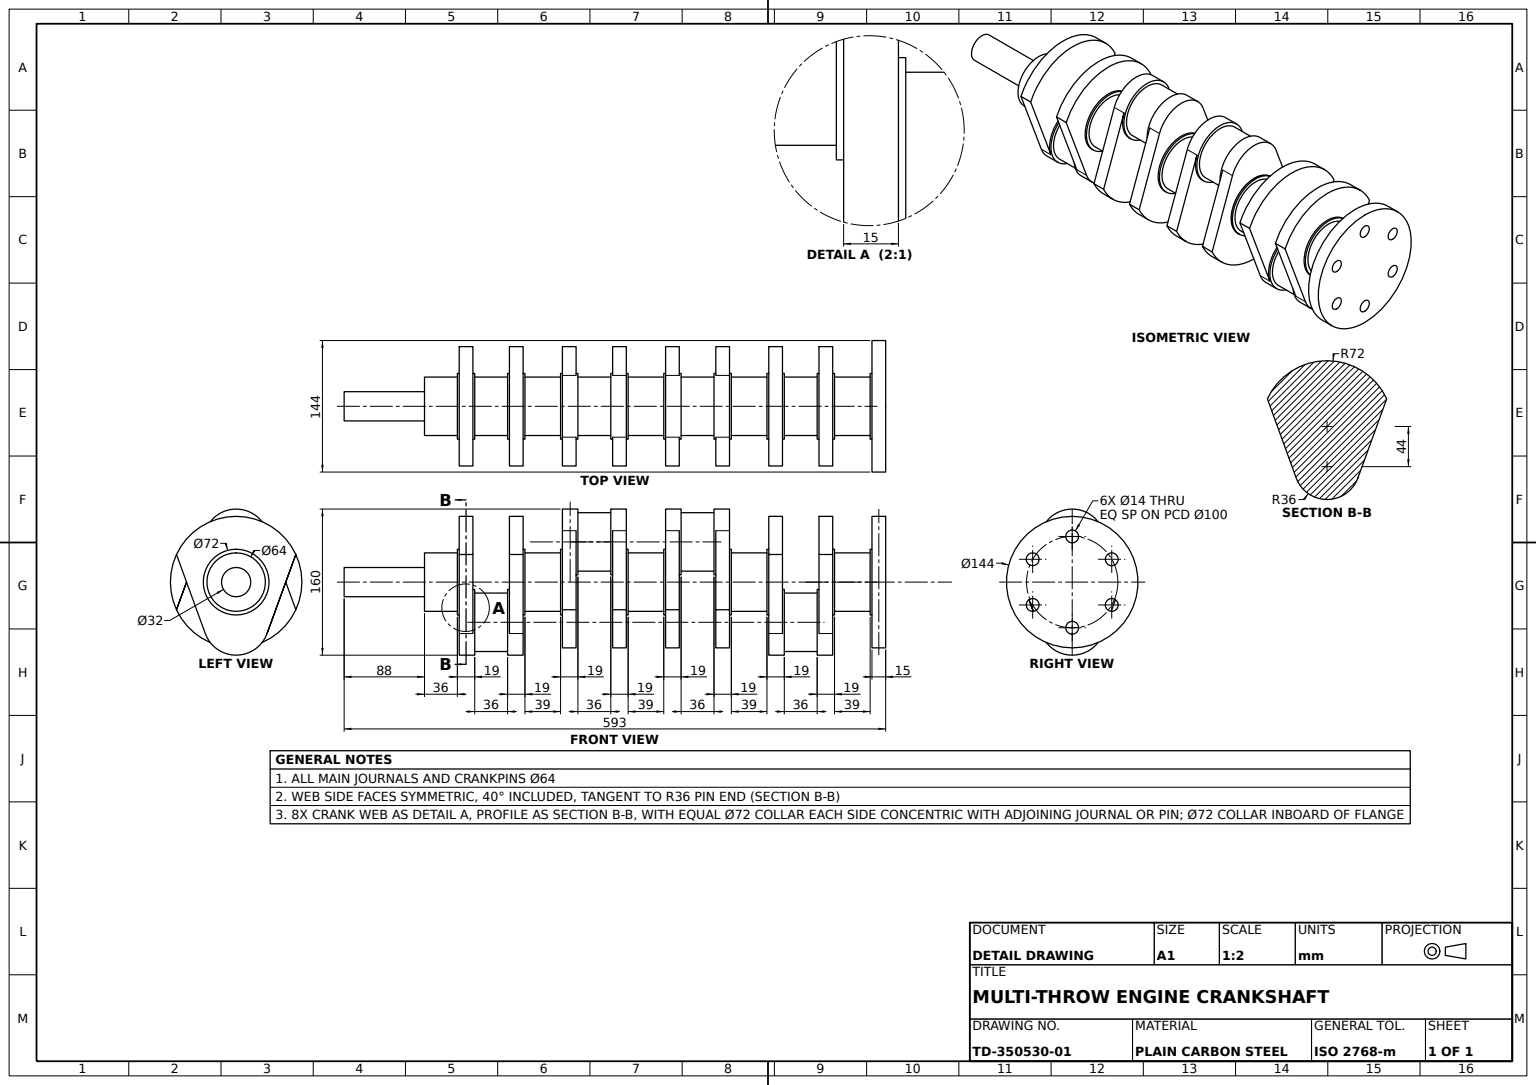
solid
v1 (111,0,36)
v2 (111,0,-36)
e1 v1 v2 CIRCLE(AX(P(111,0,0),D(-1,0,0),D(0,0,1)),36)
e2 v2 v1 CIRCLE(AX(P(111,0,0),D(-1,0,0),D(0,0,1)),36)
v3 (111,0,32)
v4 (111,0,-32)
e3 v3 v4 CIRCLE(AX(P(111,0,0),D(-1,0,0),D(0,0,1)),32)
e4 v4 v3 CIRCLE(AX(P(111,0,0),D(-1,0,0),D(0,0,1)),32)
face PLANE(AX(P(111,36,0),D(1,0,0),D(0,0,-1))) rev [e1 e2] [-e3 -e4]
v5 (452,36,0)
v6 (452,-36,0)
e5 v5 v6 CIRCLE(AX(P(452,0,0),D(1,0,0),D(0,1,0)),36)
e6 v6 v5 CIRCLE(AX(P(452,0,0),D(1,0,0),D(0,1,0)),36)
v7 (452,43,0)
v8 (452,57,0)
e7 v7 v8 CIRCLE(AX(P(452,50,0),D(-1,0,0),D(0,1,0)),7)
e8 v8 v7 CIRCLE(AX(P(452,50,0),D(-1,0,0),D(0,1,0)),7)
v9 (452,32,43.30127)
v10 (452,18,43.30127)
e9 v9 v10 CIRCLE(AX(P(452,25,43.30127),D(-1,0,0),D(0,1,0)),7)
e10 v10 v9 CIRCLE(AX(P(452,25,43.30127),D(-1,0,0),D(0,1,0)),7)
v11 (452,-57,0)
v12 (452,-43,0)
e11 v11 v12 CIRCLE(AX(P(452,-50,0),D(-1,0,0),D(0,1,0)),7)
e12 v12 v11 CIRCLE(AX(P(452,-50,0),D(-1,0,0),D(0,1,0)),7)
v13 (452,18,-43.30127)
v14 (452,32,-43.30127)
e13 v13 v14 CIRCLE(AX(P(452,25,-43.30127),D(-1,0,0),D(0,1,0)),7)
e14 v14 v13 CIRCLE(AX(P(452,25,-43.30127),D(-1,0,0),D(0,1,0)),7)
v15 (452,72,0)
v16 (452,-72,0)
e15 v15 v16 CIRCLE(AX(P(452,0,0),D(1,0,0),D(0,1,0)),72)
e16 v16 v15 CIRCLE(AX(P(452,0,0),D(1,0,0),D(0,1,0)),72)
v17 (452,-18,43.30127)
v18 (452,-32,43.30127)
e17 v17 v18 CIRCLE(AX(P(452,-25,43.30127),D(-1,0,0),D(0,1,0)),7)
e18 v18 v17 CIRCLE(AX(P(452,-25,43.30127),D(-1,0,0),D(0,1,0)),7)
v19 (452,-32,-43.30127)
v20 (452,-18,-43.30127)
e19 v19 v20 CIRCLE(AX(P(452,-25,-43.30127),D(-1,0,0),D(0,1,0)),7)
e20 v20 v19 CIRCLE(AX(P(452,-25,-43.30127),D(-1,0,0),D(0,1,0)),7)
face PLANE(AX(P(452,0,0),D(1,0,0),D(0,1,0))) rev [e5 e6] [-e7 -e8] [-e9 -e10] [-e11 -e12] [-e13 -e14] [-e15 -e16] [-e17 -e18] [-e19 -e20]
v21 (130,44,-36)
v22 (130,44,36)
e21 v21 v22 CIRCLE(AX(P(130,44,0),D(1,0,0),D(0,1,0)),36)
v23 (128,44,-36)
e22 v21 v23 LINE
v24 (128,56.312725,-33.828934)
e23 v23 v24 CIRCLE(AX(P(128,44,0),D(1,0,0),D(0,1,0)),36)
v25 (113,56.312725,-33.828934)
e24 v24 v25 LINE
v26 (113,56.312725,33.828934)
e25 v25 v26 CIRCLE(AX(P(113,44,0),D(1,0,0),D(0,0,-1)),36)
v27 (128,56.312725,33.828934)
e26 v27 v26 LINE
v28 (128,44,36)
e27 v27 v28 CIRCLE(AX(P(128,44,0),D(1,0,0),D(0,1,0)),36)
e28 v22 v28 LINE
face CYL(AX(P(128,44,0),D(-1,0,0),D(0,0,1)),36) [-e21 e22 e23 e24 e25 -e26 e27 -e28]
v29 (183,0,-36)
v30 (183,0,36)
e29 v29 v30 CIRCLE(AX(P(183,0,0),D(-1,0,0),D(0,0,1)),36)
e30 v30 v29 CIRCLE(AX(P(183,0,0),D(-1,0,0),D(0,0,1)),36)
v31 (183,-30.252318,-65.336033)
v32 (183,56.312725,-33.828934)
e31 v31 v32 LINE
v33 (183,80,0)
e32 v32 v33 CIRCLE(AX(P(183,44,0),D(1,0,0),D(0,0,-1)),36)
v34 (183,56.312725,33.828934)
e33 v33 v34 CIRCLE(AX(P(183,44,0),D(1,0,0),D(0,0,-1)),36)
v35 (183,-30.252318,65.336033)
e34 v34 v35 LINE
e35 v35 v31 CIRCLE(AX(P(183,0,0),D(1,0,0),D(0,0,-1)),72)
face PLANE(AX(P(183,44,0),D(-1,0,0),D(0,0,-1))) rev [e29 e30] [e31 e32 e33 e34 e35]
v36 (226,0,-36)
v37 (226,0,36)
e36 v36 v37 CIRCLE(AX(P(226,0,0),D(-1,0,0),D(0,0,1)),36)
v38 (224,0,36)
e37 v38 v37 LINE
v39 (224,0,-36)
e38 v39 v38 CIRCLE(AX(P(224,0,0),D(-1,0,0),D(0,0,1)),36)
e39 v39 v36 LINE
face CYL(AX(P(226,0,0),D(1,0,0),D(0,0,1)),36) [e36 -e37 -e38 e39]
v40 (241,44,36)
v41 (241,44,-36)
e40 v40 v41 CIRCLE(AX(P(241,44,0),D(1,0,0),D(0,0,-1)),36)
v42 (243,44,-36)
e41 v42 v41 LINE
v43 (243,44,36)
e42 v43 v42 CIRCLE(AX(P(243,44,0),D(1,0,0),D(0,0,-1)),36)
e43 v43 v40 LINE
face CYL(AX(P(241,44,0),D(-1,0,0),D(0,0,1)),36) [e40 -e41 -e42 e43]
v44 (168,-30.252318,65.336033)
v45 (168,-30.252318,-65.336033)
e44 v44 v45 CIRCLE(AX(P(168,0,0),D(1,0,0),D(0,0,-1)),72)
v46 (168,56.312725,33.828934)
e45 v46 v44 LINE
v47 (168,8,0)
e46 v46 v47 CIRCLE(AX(P(168,44,0),D(1,0,0),D(0,1,0)),36)
v48 (168,56.312725,-33.828934)
e47 v47 v48 CIRCLE(AX(P(168,44,0),D(1,0,0),D(0,1,0)),36)
e48 v45 v48 LINE
face PLANE(AX(P(168,44,0),D(-1,0,0),D(0,0,-1))) [-e44 -e45 e46 e47 -e48]
v49 (0,30.252318,-65.336033)
v50 (0,30.252318,65.336033)
e49 v49 v50 CIRCLE(AX(P(0,0,0),D(1,0,0),D(0,-1,0)),72)
v51 (15,30.252318,65.336033)
e50 v51 v50 LINE
v52 (15,30.252318,-65.336033)
e51 v52 v51 CIRCLE(AX(P(15,0,0),D(1,0,0),D(0,-1,0)),72)
e52 v52 v49 LINE
face CYL(AX(P(15,0,0),D(-1,0,0),D(0,-1,0)),72) [e49 -e50 -e51 e52]
v53 (241,-30.252318,65.336033)
v54 (226,-30.252318,65.336033)
e53 v53 v54 LINE
v55 (241,56.312725,33.828934)
e54 v55 v53 LINE
v56 (226,56.312725,33.828934)
e55 v55 v56 LINE
e56 v56 v54 LINE
face PLANE(AX(P(241,56.312725,33.828934),D(0,-0.342020143,-0.939692621),D(0,0.939692621,-0.342020143))) rev [-e53 -e54 e55 e56]
v57 (337,32,0)
v58 (337,-32,0)
e57 v57 v58 CIRCLE(AX(P(337,0,0),D(1,0,0),D(0,1,0)),32)
v59 (298,32,0)
e58 v59 v57 LINE
v60 (298,-32,0)
e59 v59 v60 CIRCLE(AX(P(298,0,0),D(1,0,0),D(0,1,0)),32)
e60 v60 v58 LINE
face CYL(AX(P(339,0,0),D(1,0,0),D(0,1,0)),32) [-e57 -e58 e59 e60]
v61 (55,30.252318,65.336033)
v62 (70,30.252318,65.336033)
e61 v61 v62 LINE
v63 (55,-56.312725,33.828934)
e62 v61 v63 LINE
v64 (70,-56.312725,33.828934)
e63 v63 v64 LINE
e64 v62 v64 LINE
face PLANE(AX(P(55,-56.312725,33.828934),D(0,-0.342020143,0.939692621),D(0,-0.939692621,-0.342020143))) [-e61 e62 e63 -e64]
v65 (339,-36,0)
v66 (339,36,0)
e65 v65 v66 CIRCLE(AX(P(339,0,0),D(1,0,0),D(0,1,0)),36)
e66 v66 v65 CIRCLE(AX(P(339,0,0),D(1,0,0),D(0,1,0)),36)
v67 (339,-56.312725,-33.828934)
v68 (339,30.252318,-65.336033)
e67 v67 v68 LINE
v69 (339,-80,0)
e68 v69 v67 CIRCLE(AX(P(339,-44,0),D(1,0,0),D(0,1,0)),36)
v70 (339,-56.312725,33.828934)
e69 v70 v69 CIRCLE(AX(P(339,-44,0),D(1,0,0),D(0,1,0)),36)
v71 (339,30.252318,65.336033)
e70 v71 v70 LINE
e71 v68 v71 CIRCLE(AX(P(339,0,0),D(1,0,0),D(0,1,0)),72)
face PLANE(AX(P(339,0,0),D(1,0,0),D(0,1,0))) rev [e65 e66] [-e67 -e68 -e69 -e70 -e71]
v72 (467,-18,-43.30127)
v73 (467,-32,-43.30127)
e72 v72 v73 CIRCLE(AX(P(467,-25,-43.30127),D(1,0,0),D(0,1,0)),7)
e73 v19 v73 LINE
e74 v20 v72 LINE
face CYL(AX(P(-126.001,-25,-43.30127),D(1,0,0),D(0,1,0)),7) rev [e72 -e73 e19 e74]
v74 (53,-8,0)
v75 (53,-80,0)
e75 v74 v75 CIRCLE(AX(P(53,-44,0),D(1,0,0),D(0,1,0)),36)
e76 v75 v74 CIRCLE(AX(P(53,-44,0),D(1,0,0),D(0,1,0)),36)
v76 (53,-12,0)
v77 (53,-76,0)
e77 v76 v77 CIRCLE(AX(P(53,-44,0),D(1,0,0),D(0,1,0)),32)
e78 v77 v76 CIRCLE(AX(P(53,-44,0),D(1,0,0),D(0,1,0)),32)
face PLANE(AX(P(53,-12,0),D(-1,0,0),D(0,-1,0))) [-e75 -e76] [e77 e78]
v78 (113,0,36)
v79 (113,0,-36)
e79 v78 v79 CIRCLE(AX(P(113,0,0),D(-1,0,0),D(0,0,1)),36)
e80 v79 v2 LINE
e81 v78 v1 LINE
face CYL(AX(P(70,0,0),D(-1,0,0),D(0,0,1)),36) [e79 e80 -e1 -e81]
e82 v22 v21 CIRCLE(AX(P(130,44,0),D(1,0,0),D(0,1,0)),36)
v80 (130,12,0)
v81 (130,76,0)
e83 v80 v81 CIRCLE(AX(P(130,44,0),D(1,0,0),D(0,1,0)),32)
e84 v81 v80 CIRCLE(AX(P(130,44,0),D(1,0,0),D(0,1,0)),32)
face PLANE(AX(P(130,80,0),D(1,0,0),D(0,1,0))) [e82 e21] [-e83 -e84]
v82 (-38,-32,0)
v83 (-38,32,0)
e85 v82 v83 CIRCLE(AX(P(-38,0,0),D(1,0,0),D(0,1,0)),32)
e86 v83 v82 CIRCLE(AX(P(-38,0,0),D(1,0,0),D(0,1,0)),32)
v84 (-38,-16,0)
v85 (-38,16,0)
e87 v84 v85 CIRCLE(AX(P(-38,0,0),D(1,0,0),D(0,1,0)),16)
e88 v85 v84 CIRCLE(AX(P(-38,0,0),D(1,0,0),D(0,1,0)),16)
face PLANE(AX(P(-38,16,0),D(-1,0,0),D(0,-1,0))) [-e85 -e86] [e87 e88]
v86 (354,30.252318,65.336033)
v87 (354,-56.312725,33.828934)
e89 v86 v87 LINE
v88 (354,-8,0)
e90 v88 v87 CIRCLE(AX(P(354,-44,0),D(1,0,0),D(0,1,0)),36)
v89 (354,-56.312725,-33.828934)
e91 v89 v88 CIRCLE(AX(P(354,-44,0),D(1,0,0),D(0,1,0)),36)
v90 (354,30.252318,-65.336033)
e92 v89 v90 LINE
e93 v90 v86 CIRCLE(AX(P(354,0,0),D(1,0,0),D(0,1,0)),72)
face PLANE(AX(P(354,0,0),D(1,0,0),D(0,1,0))) [e89 -e90 -e91 e92 e93]
v91 (15,-56.312725,-33.828934)
v92 (0,-56.312725,-33.828934)
e94 v91 v92 LINE
v93 (15,-8,0)
e95 v91 v93 CIRCLE(AX(P(15,-44,0),D(1,0,0),D(0,1,0)),36)
v94 (17,-8,0)
e96 v94 v93 LINE
v95 (17,-80,0)
e97 v95 v94 CIRCLE(AX(P(17,-44,0),D(1,0,0),D(0,1,0)),36)
v96 (0,-80,0)
e98 v95 v96 LINE
e99 v96 v92 CIRCLE(AX(P(0,-44,0),D(1,0,0),D(0,1,0)),36)
face CYL(AX(P(15,-44,0),D(-1,0,0),D(0,-1,0)),36) [-e94 e95 -e96 -e97 e98 e99]
v97 (281,-30.252318,-65.336033)
v98 (281,56.312725,-33.828934)
e100 v97 v98 LINE
v99 (281,-30.252318,65.336033)
e101 v99 v97 CIRCLE(AX(P(281,0,0),D(1,0,0),D(0,0,-1)),72)
v100 (281,56.312725,33.828934)
e102 v100 v99 LINE
v101 (281,44,36)
e103 v100 v101 CIRCLE(AX(P(281,44,0),D(1,0,0),D(0,0,-1)),36)
v102 (281,44,-36)
e104 v101 v102 CIRCLE(AX(P(281,44,0),D(1,0,0),D(0,0,-1)),36)
e105 v102 v98 CIRCLE(AX(P(281,44,0),D(1,0,0),D(0,0,-1)),36)
face PLANE(AX(P(281,44,0),D(-1,0,0),D(0,0,-1))) [-e100 -e101 -e102 e103 e104 e105]
v103 (337,-36,0)
v104 (337,36,0)
e106 v103 v104 CIRCLE(AX(P(337,0,0),D(1,0,0),D(0,1,0)),36)
e107 v104 v66 LINE
e108 v103 v65 LINE
face CYL(AX(P(339,0,0),D(1,0,0),D(0,1,0)),36) [e106 e107 -e65 -e108]
v105 (226,-30.252318,-65.336033)
e109 v54 v105 CIRCLE(AX(P(226,0,0),D(1,0,0),D(0,0,-1)),72)
v106 (241,-30.252318,-65.336033)
e110 v106 v105 LINE
e111 v53 v106 CIRCLE(AX(P(241,0,0),D(1,0,0),D(0,0,-1)),72)
face CYL(AX(P(241,0,0),D(-1,0,0),D(0,0,1)),72) [e109 -e110 -e111 e53]
v107 (55,-8,0)
e112 v107 v63 CIRCLE(AX(P(55,-44,0),D(1,0,0),D(0,1,0)),36)
e113 v74 v107 LINE
v108 (70,-80,0)
e114 v75 v108 LINE
e115 v64 v108 CIRCLE(AX(P(70,-44,0),D(1,0,0),D(0,1,0)),36)
face CYL(AX(P(55,-44,0),D(1,0,0),D(0,1,0)),36) [-e112 -e113 e75 e114 -e115 -e63]
e116 v89 v67 LINE
e117 v90 v68 LINE
face PLANE(AX(P(354,-56.312725,-33.828934),D(0,0.342020143,0.939692621),D(0,-0.939692621,0.342020143))) rev [-e92 e116 e67 -e117]
v109 (467,-32,43.30127)
e118 v18 v109 LINE
v110 (467,-18,43.30127)
e119 v109 v110 CIRCLE(AX(P(467,-25,43.30127),D(1,0,0),D(0,1,0)),7)
e120 v17 v110 LINE
face CYL(AX(P(-126.001,-25,43.30127),D(1,0,0),D(0,1,0)),7) rev [e17 e118 e119 -e120]
v111 (70,0,36)
v112 (70,0,-36)
e121 v111 v112 CIRCLE(AX(P(70,0,0),D(-1,0,0),D(0,0,1)),36)
e122 v112 v111 CIRCLE(AX(P(70,0,0),D(-1,0,0),D(0,0,1)),36)
v113 (70,-56.312725,-33.828934)
e123 v108 v113 CIRCLE(AX(P(70,-44,0),D(1,0,0),D(0,1,0)),36)
v114 (70,30.252318,-65.336033)
e124 v113 v114 LINE
v115 (70,72,0)
e125 v114 v115 CIRCLE(AX(P(70,0,0),D(1,0,0),D(0,-1,0)),72)
e126 v115 v62 CIRCLE(AX(P(70,0,0),D(1,0,0),D(0,-1,0)),72)
face PLANE(AX(P(70,0,0),D(1,0,0),D(0,-1,0))) [e121 e122] [e123 e124 e125 e126 e64 e115]
e127 v45 v31 LINE
e128 v48 v32 LINE
face PLANE(AX(P(168,-30.252318,-65.336033),D(0,0.342020143,-0.939692621),D(0,0.939692621,0.342020143))) [-e127 e48 e128 -e31]
e129 v28 v23 CIRCLE(AX(P(128,44,0),D(1,0,0),D(0,1,0)),36)
v116 (128,-30.252318,65.336033)
e130 v27 v116 LINE
v117 (128,-30.252318,-65.336033)
e131 v116 v117 CIRCLE(AX(P(128,0,0),D(1,0,0),D(0,0,-1)),72)
e132 v117 v24 LINE
face PLANE(AX(P(128,44,0),D(1,0,0),D(0,0,-1))) [-e129 -e27 e130 e131 e132 -e23]
v118 (411,36,0)
v119 (409,36,0)
e133 v118 v119 LINE
v120 (409,-36,0)
e134 v119 v120 CIRCLE(AX(P(409,0,0),D(1,0,0),D(0,1,0)),36)
v121 (411,-36,0)
e135 v121 v120 LINE
e136 v118 v121 CIRCLE(AX(P(411,0,0),D(1,0,0),D(0,1,0)),36)
face CYL(AX(P(409,0,0),D(-1,0,0),D(0,1,0)),36) [e133 e134 -e135 -e136]
v122 (467,18,43.30127)
e137 v10 v122 LINE
v123 (467,32,43.30127)
e138 v122 v123 CIRCLE(AX(P(467,25,43.30127),D(1,0,0),D(0,1,0)),7)
e139 v9 v123 LINE
face CYL(AX(P(-126.001,25,43.30127),D(1,0,0),D(0,1,0)),7) rev [e9 e137 e138 -e139]
v124 (394,-56.312725,33.828934)
v125 (409,-56.312725,33.828934)
e140 v124 v125 LINE
v126 (409,30.252318,65.336033)
e141 v126 v125 LINE
v127 (394,30.252318,65.336033)
e142 v127 v126 LINE
e143 v127 v124 LINE
face PLANE(AX(P(394,30.252318,65.336033),D(0,-0.342020143,0.939692621),D(0,-0.939692621,-0.342020143))) [e140 -e141 -e142 e143]
v128 (166,76,0)
e144 v81 v128 LINE
v129 (166,12,0)
e145 v80 v129 LINE
e146 v128 v129 CIRCLE(AX(P(166,44,0),D(1,0,0),D(0,1,0)),32)
face CYL(AX(P(168,44,0),D(1,0,0),D(0,1,0)),32) [-e144 e84 e145 -e146]
v130 (467,43,0)
e147 v7 v130 LINE
v131 (467,57,0)
e148 v130 v131 CIRCLE(AX(P(467,50,0),D(1,0,0),D(0,1,0)),7)
e149 v8 v131 LINE
face CYL(AX(P(-126.001,50,0),D(1,0,0),D(0,1,0)),7) rev [e147 e148 -e149 e8]
v132 (296,-36,0)
v133 (296,36,0)
e150 v132 v133 CIRCLE(AX(P(296,0,0),D(1,0,0),D(0,1,0)),36)
e151 v133 v132 CIRCLE(AX(P(296,0,0),D(1,0,0),D(0,1,0)),36)
v134 (296,56.312725,33.828934)
v135 (296,-30.252318,65.336033)
e152 v134 v135 LINE
v136 (296,-30.252318,-65.336033)
e153 v135 v136 CIRCLE(AX(P(296,0,0),D(1,0,0),D(0,0,-1)),72)
v137 (296,56.312725,-33.828934)
e154 v136 v137 LINE
e155 v137 v134 CIRCLE(AX(P(296,44,0),D(1,0,0),D(0,0,-1)),36)
face PLANE(AX(P(296,44,0),D(-1,0,0),D(0,0,-1))) rev [-e150 -e151] [e152 e153 e154 e155]
v138 (392,-76,0)
v139 (392,-12,0)
e156 v138 v139 CIRCLE(AX(P(392,-44,0),D(1,0,0),D(0,1,0)),32)
e157 v139 v138 CIRCLE(AX(P(392,-44,0),D(1,0,0),D(0,1,0)),32)
v140 (392,-80,0)
v141 (392,-8,0)
e158 v140 v141 CIRCLE(AX(P(392,-44,0),D(1,0,0),D(0,1,0)),36)
e159 v141 v140 CIRCLE(AX(P(392,-44,0),D(1,0,0),D(0,1,0)),36)
face PLANE(AX(P(392,-76,0),D(1,0,0),D(0,1,0))) rev [e156 e157] [-e158 -e159]
v142 (394,72,0)
v143 (409,72,0)
e160 v142 v143 LINE
v144 (409,30.252318,-65.336033)
e161 v144 v143 CIRCLE(AX(P(409,0,0),D(1,0,0),D(0,1,0)),72)
v145 (394,30.252318,-65.336033)
e162 v145 v144 LINE
e163 v145 v142 CIRCLE(AX(P(394,0,0),D(1,0,0),D(0,1,0)),72)
face CYL(AX(P(394,0,0),D(1,0,0),D(0,1,0)),72) [e160 -e161 -e162 e163]
v146 (-126,16,0)
v147 (-126,-16,0)
e164 v146 v147 CIRCLE(AX(P(-126,0,0),D(1,0,0),D(0,1,0)),16)
e165 v147 v84 LINE
e166 v146 v85 LINE
face CYL(AX(P(0,0,0),D(1,0,0),D(0,1,0)),16) [e164 e165 -e88 -e166]
v148 (356,-12,0)
e167 v148 v139 LINE
v149 (356,-76,0)
e168 v148 v149 CIRCLE(AX(P(356,-44,0),D(1,0,0),D(0,1,0)),32)
e169 v149 v138 LINE
face CYL(AX(P(394,-44,0),D(1,0,0),D(0,1,0)),32) [-e167 e168 e169 -e157]
v150 (298,-36,0)
e170 v132 v150 LINE
v151 (298,36,0)
e171 v133 v151 LINE
e172 v150 v151 CIRCLE(AX(P(298,0,0),D(1,0,0),D(0,1,0)),36)
face CYL(AX(P(339,0,0),D(1,0,0),D(0,1,0)),36) [-e170 e150 e171 -e172]
v152 (185,0,36)
v153 (185,0,-36)
e173 v152 v153 CIRCLE(AX(P(185,0,0),D(-1,0,0),D(0,0,1)),36)
e174 v29 v153 LINE
e175 v30 v152 LINE
face CYL(AX(P(226,0,0),D(1,0,0),D(0,0,1)),36) [e173 -e174 -e30 e175]
v154 (72,0,32)
v155 (72,0,-32)
e176 v154 v155 CIRCLE(AX(P(72,0,0),D(-1,0,0),D(0,0,1)),32)
e177 v3 v154 LINE
e178 v4 v155 LINE
face CYL(AX(P(70,0,0),D(-1,0,0),D(0,0,1)),32) [-e176 -e177 e3 e178]
v156 (279,44,36)
e179 v156 v101 LINE
v157 (279,44,-36)
e180 v156 v157 CIRCLE(AX(P(279,44,0),D(1,0,0),D(0,0,-1)),36)
e181 v157 v102 LINE
face CYL(AX(P(281,44,0),D(1,0,0),D(0,0,-1)),36) [-e179 e180 e181 -e104]
v158 (450,-32,0)
v159 (450,32,0)
e182 v158 v159 CIRCLE(AX(P(450,0,0),D(1,0,0),D(0,1,0)),32)
e183 v159 v158 CIRCLE(AX(P(450,0,0),D(1,0,0),D(0,1,0)),32)
v160 (450,-36,0)
v161 (450,36,0)
e184 v160 v161 CIRCLE(AX(P(450,0,0),D(1,0,0),D(0,1,0)),36)
e185 v161 v160 CIRCLE(AX(P(450,0,0),D(1,0,0),D(0,1,0)),36)
face PLANE(AX(P(450,36,0),D(-1,0,0),D(0,1,0))) [e182 e183] [-e184 -e185]
v162 (467,-43,0)
v163 (467,-57,0)
e186 v162 v163 CIRCLE(AX(P(467,-50,0),D(1,0,0),D(0,1,0)),7)
e187 v11 v163 LINE
e188 v12 v162 LINE
face CYL(AX(P(-126.001,-50,0),D(1,0,0),D(0,1,0)),7) rev [e186 -e187 e11 e188]
e189 v110 v109 CIRCLE(AX(P(467,-25,43.30127),D(1,0,0),D(0,1,0)),7)
face CYL(AX(P(-126.001,-25,43.30127),D(1,0,0),D(0,1,0)),7) rev [e189 -e118 e18 e120]
e190 v6 v160 LINE
e191 v5 v161 LINE
face CYL(AX(P(409,0,0),D(-1,0,0),D(0,1,0)),36) [-e190 -e5 e191 e185]
v164 (166,8,0)
e192 v164 v47 LINE
v165 (166,80,0)
e193 v164 v165 CIRCLE(AX(P(166,44,0),D(1,0,0),D(0,1,0)),36)
e194 v165 v33 LINE
face CYL(AX(P(168,44,0),D(1,0,0),D(0,1,0)),36) [-e47 -e192 e193 e194 -e32 -e128]
v166 (113,-30.252318,65.336033)
v167 (113,-30.252318,-65.336033)
e195 v166 v167 CIRCLE(AX(P(113,0,0),D(1,0,0),D(0,0,-1)),72)
e196 v26 v166 LINE
e197 v167 v25 LINE
e198 v79 v78 CIRCLE(AX(P(113,0,0),D(-1,0,0),D(0,0,1)),36)
face PLANE(AX(P(113,44,0),D(1,0,0),D(0,0,-1))) rev [-e195 -e196 -e25 -e197] [-e79 -e198]
v168 (409,-56.312725,-33.828934)
e199 v168 v144 LINE
v169 (394,-56.312725,-33.828934)
e200 v169 v168 LINE
e201 v169 v145 LINE
face PLANE(AX(P(394,-56.312725,-33.828934),D(0,-0.342020143,-0.939692621),D(0,0.939692621,-0.342020143))) [e162 -e199 -e200 e201]
e202 v151 v150 CIRCLE(AX(P(298,0,0),D(1,0,0),D(0,1,0)),36)
face CYL(AX(P(339,0,0),D(1,0,0),D(0,1,0)),36) [e151 e170 -e202 -e171]
e203 v116 v166 LINE
e204 v117 v167 LINE
face CYL(AX(P(128,0,0),D(-1,0,0),D(0,0,1)),72) [-e131 e203 e195 -e204]
v170 (241,56.312725,-33.828934)
e205 v41 v170 CIRCLE(AX(P(241,44,0),D(1,0,0),D(0,0,-1)),36)
v171 (226,56.312725,-33.828934)
e206 v170 v171 LINE
e207 v171 v56 CIRCLE(AX(P(226,44,0),D(1,0,0),D(0,0,-1)),36)
e208 v55 v40 CIRCLE(AX(P(241,44,0),D(1,0,0),D(0,0,-1)),36)
e209 v42 v43 CIRCLE(AX(P(243,44,0),D(1,0,0),D(0,0,-1)),36)
face CYL(AX(P(241,44,0),D(-1,0,0),D(0,0,1)),36) [e205 e206 e207 -e55 e208 -e43 -e209 e41]
e210 v106 v170 LINE
face PLANE(AX(P(241,44,0),D(1,0,0),D(0,0,-1))) [-e208 e54 e111 e210 -e205 -e40]
face PLANE(AX(P(128,56.312725,33.828934),D(0,-0.342020143,-0.939692621),D(0,0.939692621,-0.342020143))) rev [-e203 -e130 e26 e196]
e211 v38 v39 CIRCLE(AX(P(224,0,0),D(-1,0,0),D(0,0,1)),36)
e212 v37 v36 CIRCLE(AX(P(226,0,0),D(-1,0,0),D(0,0,1)),36)
face CYL(AX(P(226,0,0),D(1,0,0),D(0,0,1)),36) [-e39 -e211 e37 e212]
v172 (55,72,0)
e213 v172 v61 CIRCLE(AX(P(55,0,0),D(1,0,0),D(0,-1,0)),72)
v173 (55,30.252318,-65.336033)
e214 v173 v172 CIRCLE(AX(P(55,0,0),D(1,0,0),D(0,-1,0)),72)
v174 (55,-56.312725,-33.828934)
e215 v174 v173 LINE
e216 v174 v107 CIRCLE(AX(P(55,-44,0),D(1,0,0),D(0,1,0)),36)
face PLANE(AX(P(55,0,0),D(1,0,0),D(0,-1,0))) rev [-e213 -e214 -e215 e216 e112 -e62]
e217 v174 v113 LINE
e218 v173 v114 LINE
face PLANE(AX(P(55,-56.312725,-33.828934),D(0,-0.342020143,-0.939692621),D(0,0.939692621,-0.342020143))) [-e124 -e217 e215 e218]
e219 v104 v103 CIRCLE(AX(P(337,0,0),D(1,0,0),D(0,1,0)),36)
face CYL(AX(P(339,0,0),D(1,0,0),D(0,1,0)),36) [e108 -e66 -e107 e219]
v175 (0,36,0)
v176 (0,-36,0)
e220 v175 v176 CIRCLE(AX(P(0,0,0),D(1,0,0),D(0,1,0)),36)
e221 v176 v175 CIRCLE(AX(P(0,0,0),D(1,0,0),D(0,1,0)),36)
v177 (0,-56.312725,33.828934)
e222 v177 v96 CIRCLE(AX(P(0,-44,0),D(1,0,0),D(0,1,0)),36)
e223 v50 v177 LINE
e224 v92 v49 LINE
face PLANE(AX(P(0,0,0),D(-1,0,0),D(0,-1,0))) [e220 e221] [-e99 -e222 -e223 -e49 -e224]
e225 v153 v152 CIRCLE(AX(P(185,0,0),D(-1,0,0),D(0,0,1)),36)
face CYL(AX(P(226,0,0),D(1,0,0),D(0,0,1)),36) [e225 -e175 -e29 e174]
e226 v97 v136 LINE
e227 v99 v135 LINE
face CYL(AX(P(281,0,0),D(1,0,0),D(0,0,-1)),72) [e226 -e153 -e227 e101]
e228 v121 v118 CIRCLE(AX(P(411,0,0),D(1,0,0),D(0,1,0)),36)
v178 (411,32,0)
v179 (411,-32,0)
e229 v178 v179 CIRCLE(AX(P(411,0,0),D(1,0,0),D(0,1,0)),32)
e230 v179 v178 CIRCLE(AX(P(411,0,0),D(1,0,0),D(0,1,0)),32)
face PLANE(AX(P(411,32,0),D(1,0,0),D(0,-1,0))) [e136 e228] [-e229 -e230]
face CYL(AX(P(55,-44,0),D(1,0,0),D(0,1,0)),36) [-e123 -e114 e76 e113 -e216 e217]
v180 (224,0,-32)
v181 (224,0,32)
e231 v180 v181 CIRCLE(AX(P(224,0,0),D(-1,0,0),D(0,0,1)),32)
e232 v181 v180 CIRCLE(AX(P(224,0,0),D(-1,0,0),D(0,0,1)),32)
face PLANE(AX(P(224,32,0),D(1,0,0),D(0,0,1))) rev [e38 e211] [-e231 -e232]
v182 (467,72,0)
e233 v182 v15 LINE
v183 (467,-72,0)
e234 v183 v182 CIRCLE(AX(P(467,0,0),D(1,0,0),D(0,1,0)),72)
e235 v183 v16 LINE
face CYL(AX(P(467,0,0),D(-1,0,0),D(0,-1,0)),72) [e16 -e233 -e234 e235]
v184 (72,0,36)
e236 v184 v111 LINE
v185 (72,0,-36)
e237 v184 v185 CIRCLE(AX(P(72,0,0),D(-1,0,0),D(0,0,1)),36)
e238 v185 v112 LINE
face CYL(AX(P(70,0,0),D(-1,0,0),D(0,0,1)),36) [-e236 e237 e238 -e121]
v186 (15,-56.312725,33.828934)
e239 v186 v177 LINE
e240 v51 v186 LINE
face PLANE(AX(P(15,-56.312725,33.828934),D(0,0.342020143,-0.939692621),D(0,0.939692621,0.342020143))) rev [-e239 -e240 e50 e223]
v187 (243,44,32)
v188 (243,44,-32)
e241 v187 v188 CIRCLE(AX(P(243,44,0),D(1,0,0),D(0,0,-1)),32)
e242 v188 v187 CIRCLE(AX(P(243,44,0),D(1,0,0),D(0,0,-1)),32)
face PLANE(AX(P(243,80,0),D(1,0,0),D(0,0,-1))) [e209 e42] [-e241 -e242]
e243 v147 v146 CIRCLE(AX(P(-126,0,0),D(1,0,0),D(0,1,0)),16)
face PLANE(AX(P(-126,0,0),D(-1,0,0),D(0,-1,0))) [-e164 -e243]
e244 v91 v52 LINE
face PLANE(AX(P(15,-56.312725,-33.828934),D(0,0.342020143,0.939692621),D(0,-0.939692621,0.342020143))) rev [e94 e224 -e52 -e244]
e245 v163 v162 CIRCLE(AX(P(467,-50,0),D(1,0,0),D(0,1,0)),7)
face CYL(AX(P(-126.001,-50,0),D(1,0,0),D(0,1,0)),7) rev [e245 -e188 e12 e187]
v189 (394,-8,0)
e246 v189 v124 CIRCLE(AX(P(394,-44,0),D(1,0,0),D(0,1,0)),36)
e247 v142 v127 CIRCLE(AX(P(394,0,0),D(1,0,0),D(0,1,0)),72)
e248 v169 v189 CIRCLE(AX(P(394,-44,0),D(1,0,0),D(0,1,0)),36)
face PLANE(AX(P(394,0,0),D(-1,0,0),D(0,1,0))) [e246 -e143 -e247 -e163 -e201 e248]
e249 v120 v119 CIRCLE(AX(P(409,0,0),D(1,0,0),D(0,1,0)),36)
face CYL(AX(P(409,0,0),D(-1,0,0),D(0,1,0)),36) [e135 e249 -e133 -e228]
e250 v100 v134 LINE
e251 v98 v137 LINE
e252 v157 v156 CIRCLE(AX(P(279,44,0),D(1,0,0),D(0,0,-1)),36)
face CYL(AX(P(281,44,0),D(1,0,0),D(0,0,-1)),36) [e179 -e103 e250 -e155 -e251 -e105 -e181 e252]
e253 v159 v178 LINE
e254 v158 v179 LINE
face CYL(AX(P(409,0,0),D(-1,0,0),D(0,1,0)),32) [-e183 e253 e229 -e254]
e255 v44 v35 LINE
e256 v46 v34 LINE
face PLANE(AX(P(168,56.312725,33.828934),D(0,0.342020143,0.939692621),D(0,-0.939692621,0.342020143))) [e45 e255 -e34 -e256]
v190 (17,-76,0)
e257 v190 v77 LINE
v191 (17,-12,0)
e258 v190 v191 CIRCLE(AX(P(17,-44,0),D(1,0,0),D(0,1,0)),32)
e259 v191 v76 LINE
face CYL(AX(P(55,-44,0),D(1,0,0),D(0,1,0)),32) [-e78 -e257 e258 e259]
e260 v191 v190 CIRCLE(AX(P(17,-44,0),D(1,0,0),D(0,1,0)),32)
face CYL(AX(P(55,-44,0),D(1,0,0),D(0,1,0)),32) [-e259 e260 e257 -e77]
e261 v143 v126 CIRCLE(AX(P(409,0,0),D(1,0,0),D(0,1,0)),72)
face CYL(AX(P(394,0,0),D(1,0,0),D(0,1,0)),72) [-e261 -e160 e247 e142]
v192 (409,-80,0)
e262 v192 v168 CIRCLE(AX(P(409,-44,0),D(1,0,0),D(0,1,0)),36)
e263 v140 v192 LINE
e264 v141 v189 LINE
face CYL(AX(P(394,-44,0),D(1,0,0),D(0,1,0)),36) [e200 -e262 -e263 e158 e264 -e248]
v193 (-2,36,0)
e265 v193 v175 LINE
v194 (-2,-36,0)
e266 v193 v194 CIRCLE(AX(P(-2,0,0),D(1,0,0),D(0,1,0)),36)
e267 v194 v176 LINE
face CYL(AX(P(0,0,0),D(1,0,0),D(0,1,0)),36) [-e265 e266 e267 -e220]
v195 (279,44,32)
v196 (279,44,-32)
e268 v195 v196 CIRCLE(AX(P(279,44,0),D(1,0,0),D(0,0,-1)),32)
e269 v187 v195 LINE
e270 v188 v196 LINE
face CYL(AX(P(281,44,0),D(1,0,0),D(0,0,-1)),32) [-e268 -e269 e241 e270]
face CYL(AX(P(128,44,0),D(-1,0,0),D(0,0,1)),36) [-e82 e28 e129 -e22]
e271 v60 v59 CIRCLE(AX(P(298,0,0),D(1,0,0),D(0,1,0)),32)
face PLANE(AX(P(298,36,0),D(1,0,0),D(0,1,0))) [e202 e172] [-e271 -e59]
e272 v129 v128 CIRCLE(AX(P(166,44,0),D(1,0,0),D(0,1,0)),32)
face CYL(AX(P(168,44,0),D(1,0,0),D(0,1,0)),32) [e144 -e272 -e145 e83]
e273 v196 v195 CIRCLE(AX(P(279,44,0),D(1,0,0),D(0,0,-1)),32)
face PLANE(AX(P(279,76,0),D(-1,0,0),D(0,0,1))) [-e252 -e180] [e273 e268]
e274 v125 v192 CIRCLE(AX(P(409,-44,0),D(1,0,0),D(0,1,0)),36)
face CYL(AX(P(394,-44,0),D(1,0,0),D(0,1,0)),36) [-e264 e159 e263 -e274 -e140 -e246]
e275 v172 v115 LINE
face CYL(AX(P(55,0,0),D(1,0,0),D(0,1,0)),72) [e61 -e126 -e275 e213]
face CYL(AX(P(409,0,0),D(-1,0,0),D(0,1,0)),32) [e254 e230 -e253 -e182]
e276 v93 v186 CIRCLE(AX(P(15,-44,0),D(1,0,0),D(0,1,0)),36)
face PLANE(AX(P(15,0,0),D(-1,0,0),D(0,-1,0))) rev [-e276 -e95 e244 e51 e240]
v197 (467,32,-43.30127)
e277 v14 v197 LINE
v198 (467,18,-43.30127)
e278 v197 v198 CIRCLE(AX(P(467,25,-43.30127),D(1,0,0),D(0,1,0)),7)
e279 v13 v198 LINE
face CYL(AX(P(-126.001,25,-43.30127),D(1,0,0),D(0,1,0)),7) rev [e277 e278 -e279 e13]
face CYL(AX(P(0,0,0),D(1,0,0),D(0,1,0)),16) [e243 e166 -e87 -e165]
e280 v165 v164 CIRCLE(AX(P(166,44,0),D(1,0,0),D(0,1,0)),36)
face PLANE(AX(P(166,76,0),D(-1,0,0),D(0,-1,0))) [e146 e272] [-e193 -e280]
e281 v94 v95 CIRCLE(AX(P(17,-44,0),D(1,0,0),D(0,1,0)),36)
face CYL(AX(P(15,-44,0),D(-1,0,0),D(0,-1,0)),36) [e96 e276 e239 e222 -e98 -e281]
e282 v86 v71 LINE
face CYL(AX(P(354,0,0),D(-1,0,0),D(0,-1,0)),72) [e71 -e282 -e93 e117]
face CYL(AX(P(70,0,0),D(-1,0,0),D(0,0,1)),36) [e198 e81 -e2 -e80]
e283 v87 v70 LINE
face PLANE(AX(P(354,30.252318,65.336033),D(0,0.342020143,-0.939692621),D(0,0.939692621,0.342020143))) rev [-e283 -e89 e282 e70]
face PLANE(AX(P(17,-8,0),D(1,0,0),D(0,1,0))) [e97 e281] [-e258 -e260]
v199 (-2,32,0)
v200 (-2,-32,0)
e284 v199 v200 CIRCLE(AX(P(-2,0,0),D(1,0,0),D(0,1,0)),32)
e285 v200 v199 CIRCLE(AX(P(-2,0,0),D(1,0,0),D(0,1,0)),32)
e286 v194 v193 CIRCLE(AX(P(-2,0,0),D(1,0,0),D(0,1,0)),36)
face PLANE(AX(P(-2,32,0),D(-1,0,0),D(0,-1,0))) [e284 e285] [-e286 -e266]
face PLANE(AX(P(281,56.312725,33.828934),D(0,0.342020143,0.939692621),D(0,-0.939692621,0.342020143))) [e227 -e152 -e250 e102]
e287 v182 v183 CIRCLE(AX(P(467,0,0),D(1,0,0),D(0,1,0)),72)
e288 v131 v130 CIRCLE(AX(P(467,50,0),D(1,0,0),D(0,1,0)),7)
e289 v123 v122 CIRCLE(AX(P(467,25,43.30127),D(1,0,0),D(0,1,0)),7)
e290 v198 v197 CIRCLE(AX(P(467,25,-43.30127),D(1,0,0),D(0,1,0)),7)
e291 v73 v72 CIRCLE(AX(P(467,-25,-43.30127),D(1,0,0),D(0,1,0)),7)
face PLANE(AX(P(467,0,0),D(1,0,0),D(0,1,0))) [e234 e287] [-e288 -e148] [-e289 -e138] [-e186 -e245] [-e290 -e278] [-e189 -e119] [-e72 -e291]
e292 v58 v57 CIRCLE(AX(P(337,0,0),D(1,0,0),D(0,1,0)),32)
face CYL(AX(P(339,0,0),D(1,0,0),D(0,1,0)),32) [e271 e58 -e292 -e60]
face CYL(AX(P(-126.001,25,-43.30127),D(1,0,0),D(0,1,0)),7) rev [e14 e279 e290 -e277]
face PLANE(AX(P(128,-30.252318,-65.336033),D(0,-0.342020143,0.939692621),D(0,-0.939692621,-0.342020143))) rev [e204 e197 -e24 -e132]
face CYL(AX(P(-126.001,50,0),D(1,0,0),D(0,1,0)),7) rev [e7 e149 e288 -e147]
v201 (356,-80,0)
v202 (356,-8,0)
e293 v201 v202 CIRCLE(AX(P(356,-44,0),D(1,0,0),D(0,1,0)),36)
e294 v202 v201 CIRCLE(AX(P(356,-44,0),D(1,0,0),D(0,1,0)),36)
e295 v149 v148 CIRCLE(AX(P(356,-44,0),D(1,0,0),D(0,1,0)),32)
face PLANE(AX(P(356,-80,0),D(-1,0,0),D(0,-1,0))) rev [e293 e294] [-e168 -e295]
face PLANE(AX(P(281,-30.252318,-65.336033),D(0,0.342020143,-0.939692621),D(0,0.939692621,0.342020143))) [-e154 -e226 e100 e251]
e296 v105 v171 LINE
face PLANE(AX(P(226,44,0),D(1,0,0),D(0,0,-1))) rev [-e212 -e36] [-e56 -e207 -e296 -e109]
face PLANE(AX(P(241,-30.252318,-65.336033),D(0,-0.342020143,0.939692621),D(0,-0.939692621,-0.342020143))) rev [-e210 e110 e296 -e206]
e297 v155 v154 CIRCLE(AX(P(72,0,0),D(-1,0,0),D(0,0,1)),32)
face CYL(AX(P(70,0,0),D(-1,0,0),D(0,0,1)),32) [-e178 e4 e177 -e297]
face CYL(AX(P(-126.001,-25,-43.30127),D(1,0,0),D(0,1,0)),7) rev [e291 -e74 e20 e73]
face PLANE(AX(P(337,32,0),D(-1,0,0),D(0,-1,0))) [-e219 -e106] [e292 e57]
face CYL(AX(P(394,-44,0),D(1,0,0),D(0,1,0)),32) [e167 -e156 -e169 e295]
e298 v201 v69 LINE
e299 v202 v88 LINE
face CYL(AX(P(354,-44,0),D(-1,0,0),D(0,-1,0)),36) [-e293 e298 e68 -e116 e91 -e299]
face CYL(AX(P(168,44,0),D(1,0,0),D(0,1,0)),36) [e192 -e46 e256 -e33 -e194 e280]
face CYL(AX(P(354,-44,0),D(-1,0,0),D(0,-1,0)),36) [-e294 e299 e90 e283 e69 -e298]
face CYL(AX(P(-126.001,25,43.30127),D(1,0,0),D(0,1,0)),7) rev [e289 -e137 e10 e139]
face CYL(AX(P(281,44,0),D(1,0,0),D(0,0,-1)),32) [-e273 -e270 e242 e269]
v203 (185,0,32)
v204 (185,0,-32)
e300 v203 v204 CIRCLE(AX(P(185,0,0),D(-1,0,0),D(0,0,1)),32)
e301 v203 v181 LINE
e302 v204 v180 LINE
face CYL(AX(P(226,0,0),D(1,0,0),D(0,0,1)),32) [-e300 e301 e232 -e302]
e303 v83 v199 LINE
e304 v82 v200 LINE
face CYL(AX(P(0,0,0),D(1,0,0),D(0,1,0)),32) [-e284 -e303 e86 e304]
e305 v185 v184 CIRCLE(AX(P(72,0,0),D(-1,0,0),D(0,0,1)),36)
face PLANE(AX(P(72,32,0),D(-1,0,0),D(0,0,1))) rev [-e305 -e237] [e176 e297]
face CYL(AX(P(70,0,0),D(-1,0,0),D(0,0,1)),36) [e305 e236 -e122 -e238]
face CYL(AX(P(55,0,0),D(1,0,0),D(0,1,0)),72) [e275 -e125 -e218 e214]
e306 v204 v203 CIRCLE(AX(P(185,0,0),D(-1,0,0),D(0,0,1)),32)
face CYL(AX(P(226,0,0),D(1,0,0),D(0,0,1)),32) [e302 e231 -e301 -e306]
face PLANE(AX(P(185,36,0),D(-1,0,0),D(0,0,-1))) rev [e306 e300] [-e225 -e173]
face CYL(AX(P(409,0,0),D(-1,0,0),D(0,1,0)),36) [e184 -e191 -e6 e190]
face PLANE(AX(P(409,0,0),D(-1,0,0),D(0,1,0))) rev [e274 e262 e199 e161 e261 e141] [-e134 -e249]
face CYL(AX(P(0,0,0),D(1,0,0),D(0,1,0)),32) [-e304 e85 e303 -e285]
face CYL(AX(P(0,0,0),D(1,0,0),D(0,1,0)),36) [-e267 e286 e265 -e221]
face CYL(AX(P(467,0,0),D(-1,0,0),D(0,-1,0)),72) [e15 -e235 -e287 e233]
face CYL(AX(P(168,0,0),D(1,0,0),D(0,0,-1)),72) [e44 e127 -e35 -e255]
